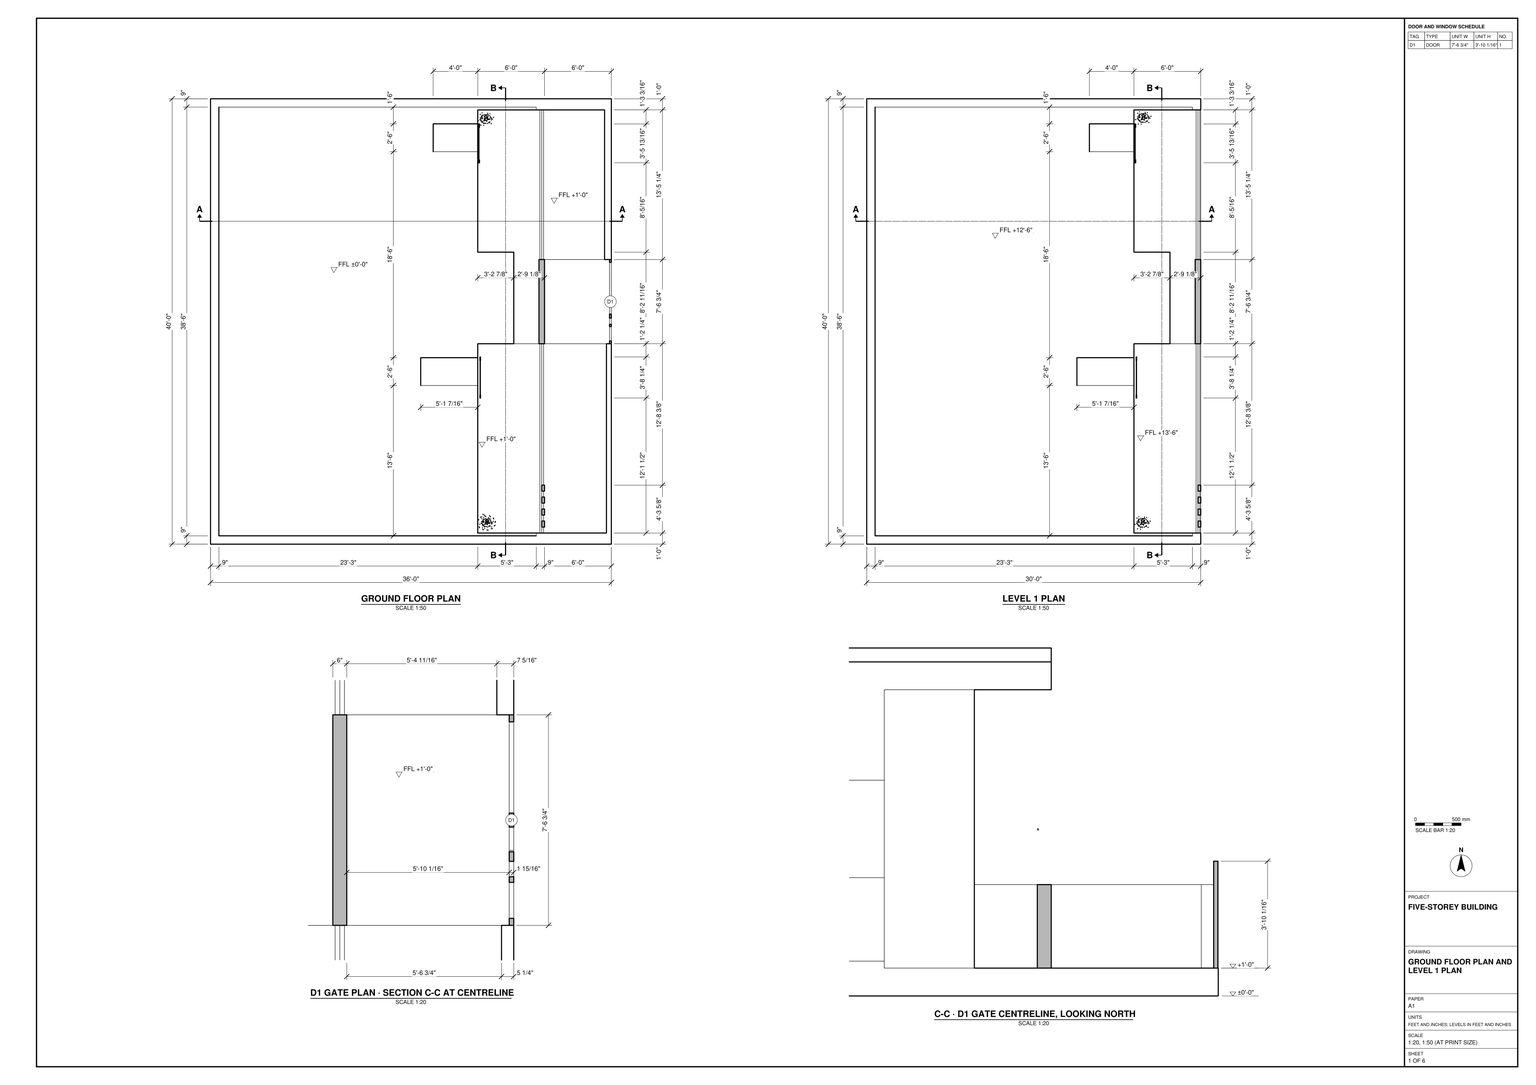
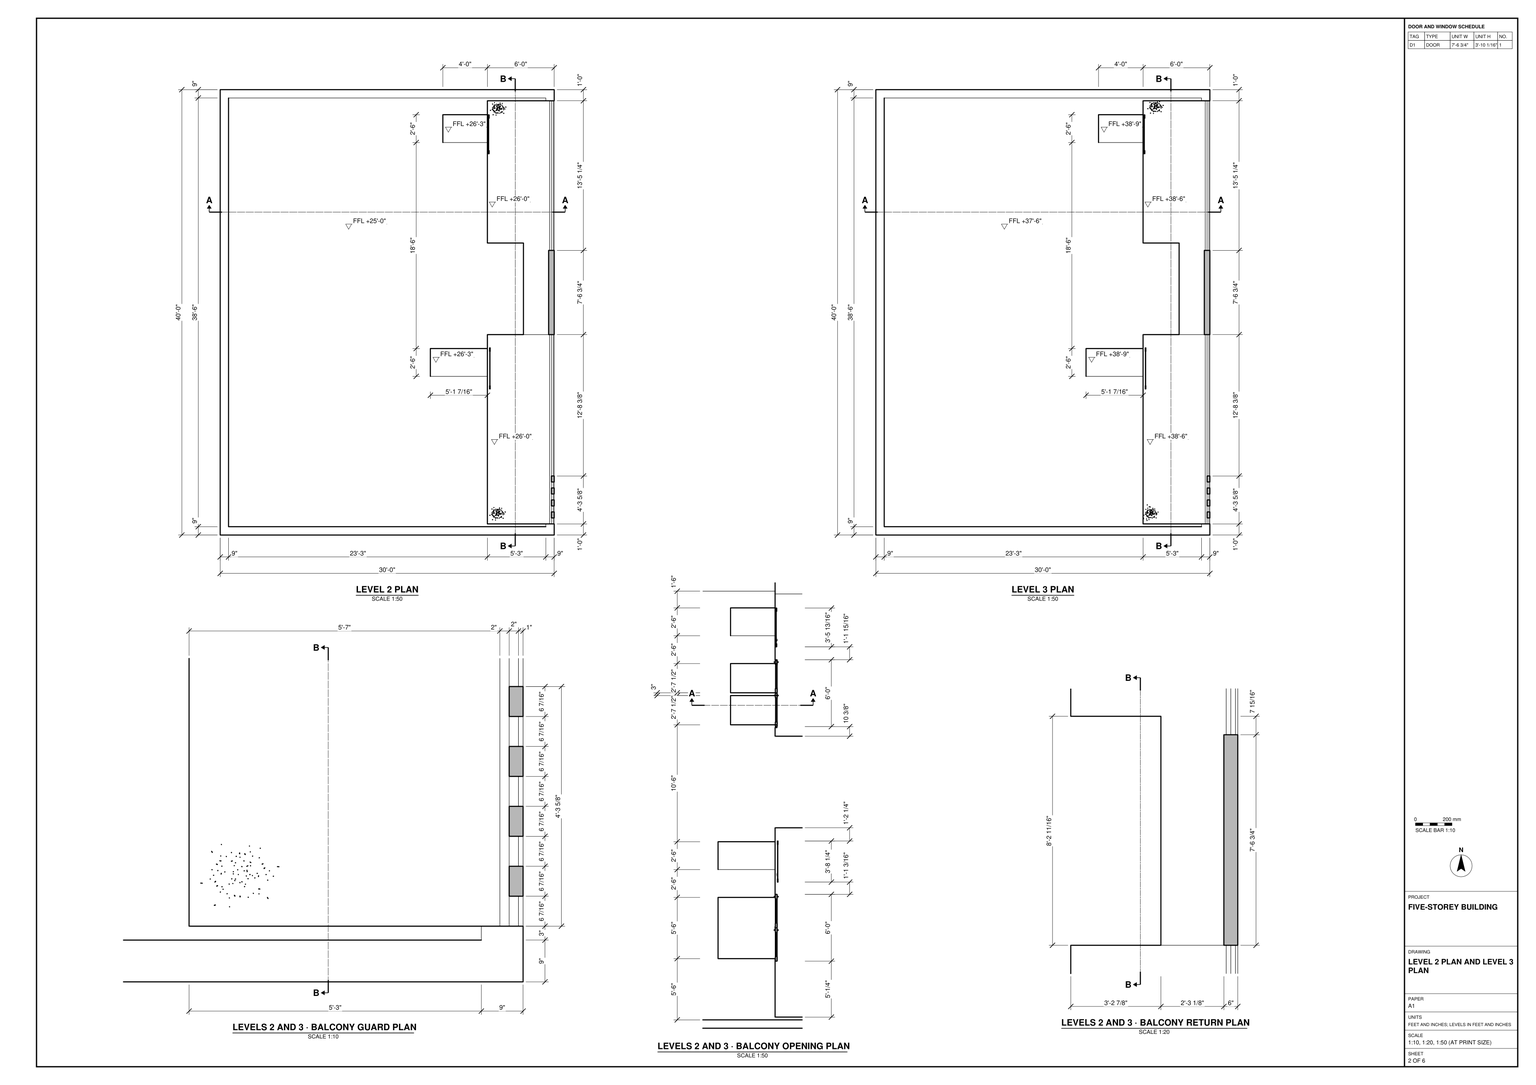
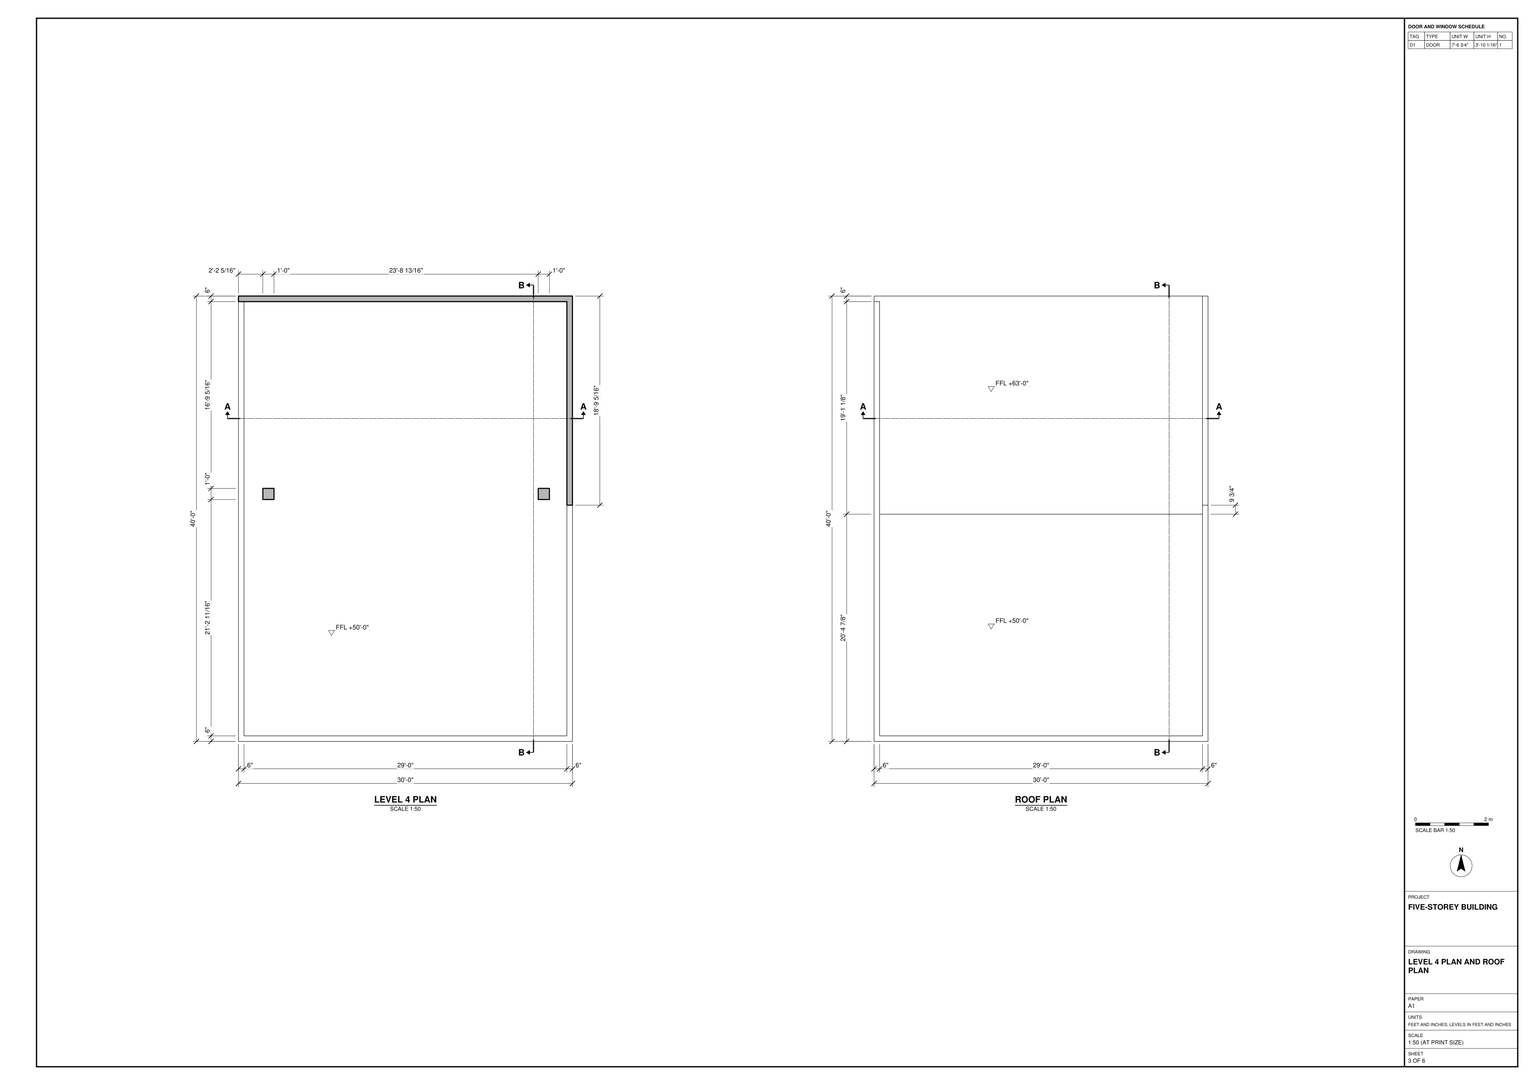
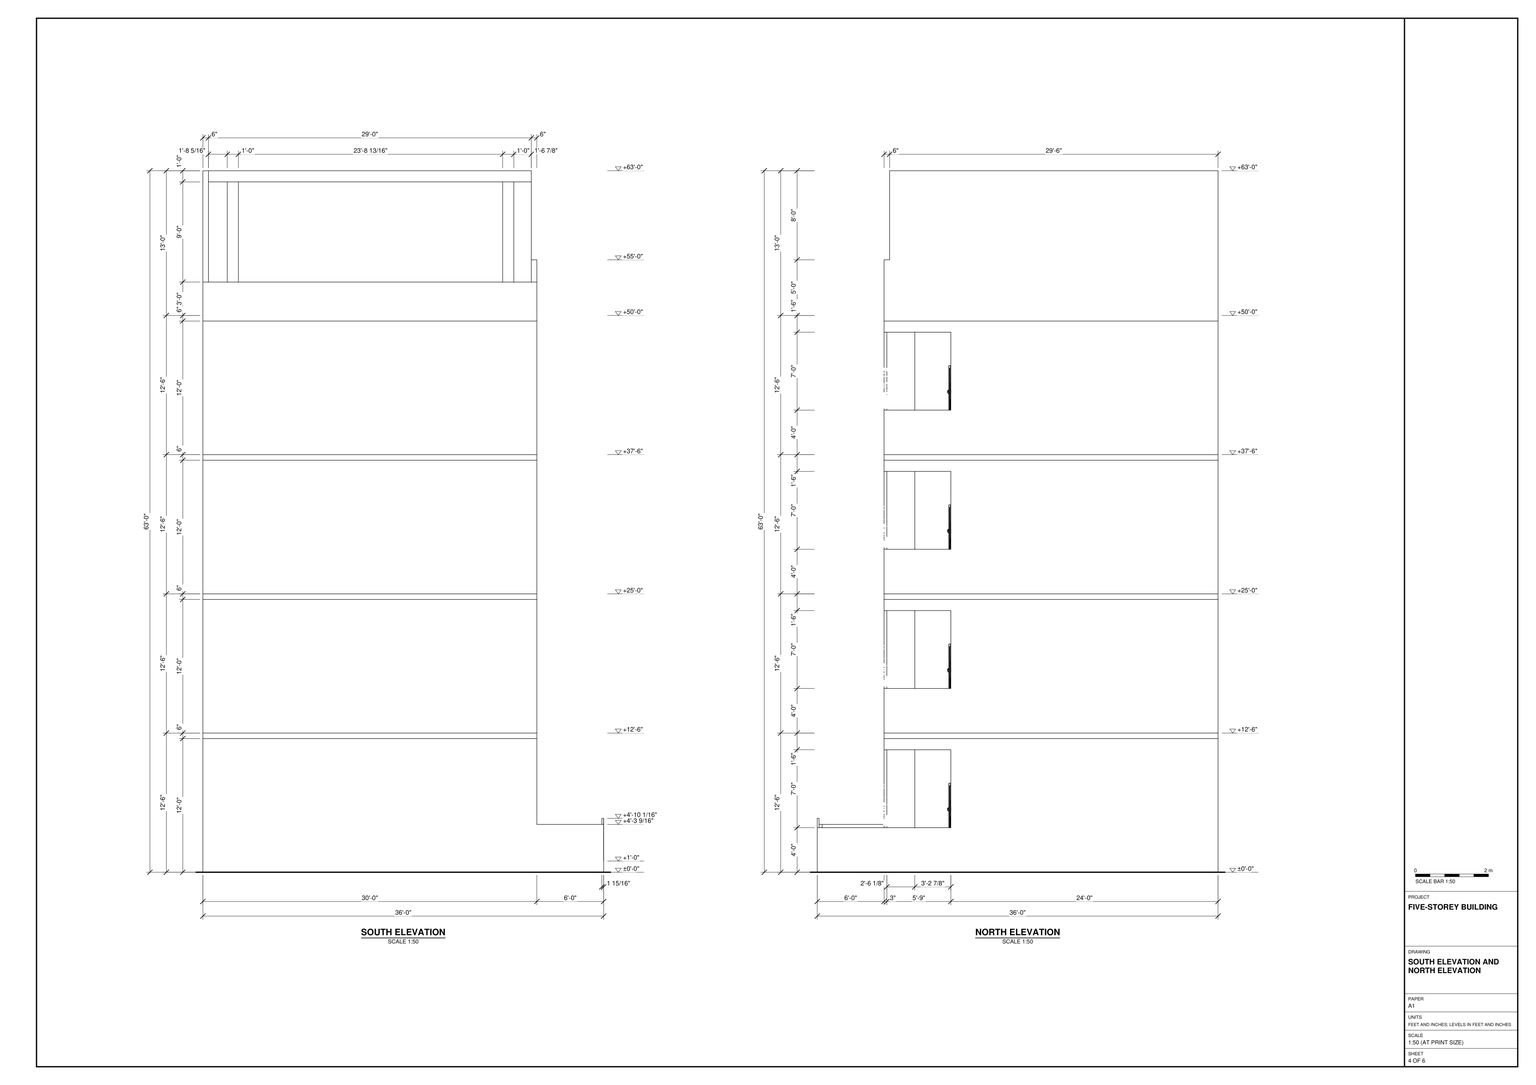
Build the five-storey building in SketchUp from task_files/diagram_01.pdf. Work in feet and inches. The model measures 36'-0" along X, 40'-0" along Y and 63'-0" in height. Set the storey levels to ±0'-0", +12'-6", +25'-0", +37'-6" and +50'-0".

Lay out the rectangular ground floor with the raised strip along its east edge. Fit the entrance gate in the break in the outer wall of this strip, using the gate plan and section for its size and position. Set the upper floors back from the gate side to give them a width of 30'-0" while retaining the full depth. Model the floor slabs, wall thicknesses and openings as drawn. Follow the balcony plans for the changes in floor height, the wider end portions and the narrow connecting portion. Include the guard members, returns and planting at the ends shown on the plans.

At +50'-0", distinguish the open terrace from the portion under the higher roof. Model the perimeter edges, walls and square supports in their drawn positions. Decor and loose items, including plants, may be any suitable library components.

Keep the walls, slabs and roof as separate groups or components, and group each furniture or joinery piece separately where shown. Use components for repeated parts. Save one SketchUp model as output_files/five_storey_building_stepped_balconies_and_roof_terrace.skp.

# SketchUp Ruby script. Lengths in inches.
U = 1.inch
M = Sketchup.active_model
def pt(a) = Geom::Point3d.new(a.map { |v| v * U })
def face(e, loops, mat)
  f = e.add_face(loops[0].map { |a| pt(a) })
  loops[1..].each { |l| e.add_face(l.map { |a| pt(a) }).erase! }
  f.material = f.back_material = mat if mat
  f
end
# faces: each face lists its corners as indices into pts; further lists are holes
def faces(e, pts, list, mat = nil) = list.each { |f| face(e, (f[0].is_a?(Array) ? f : [f]).map { |l| l.map { |i| pts[i] } }, mat) }
# xy, xz, yz: faces in a plane at the given z, y or x. An outline is a flat list of corners, or four numbers for a rectangle; further outlines are holes
def ring(l) = l.size == 4 ? [[l[0], l[1]], [l[2], l[1]], [l[2], l[3]], [l[0], l[3]]] : l.each_slice(2).to_a
def flat(e, list, mat, &to3) = list.each { |f| face(e, (f[0].is_a?(Array) ? f : [f]).map { |l| ring(l).map { |u, v| to3.(u, v) } }, mat) }
def xy(e, z, list, mat = nil) = flat(e, list, mat) { |x, y| [x, y, z] }
def xz(e, y, list, mat = nil) = flat(e, list, mat) { |x, z| [x, y, z] }
def yz(e, x, list, mat = nil) = flat(e, list, mat) { |y, z| [x, y, z] }
def lines(e, pts, list) = list.each { |a, b| e.add_line(pt(pts[a]), pt(pts[b])) }
# prism: a flat outline (further loops are holes) pulled along v
def prism(e, loops, v, mat = nil)
  f = face(e, loops, mat); d = Geom::Vector3d.new(v.map { |x| x * U })
  f.pushpull(f.normal.samedirection?(d) ? d.length : -d.length)
end
def box(e, o, s, mat = nil) = prism(e, [[o, [o[0] + s[0], o[1], o[2]], [o[0] + s[0], o[1] + s[1], o[2]], [o[0], o[1] + s[1], o[2]]]], [0, 0, s[2]], mat)
def at(x, y, z, deg = 0) = Geom::Transformation.translation(pt([x, y, z])) * Geom::Transformation.rotation(ORIGIN, Z_AXIS, deg.degrees)
def axes(o, x, y, z) = Geom::Transformation.new([*x, 0, *y, 0, *z, 0, *pt(o).to_a, 1])
def part(name) = M.definitions.add(name)
# library, detail: a bought-in or finely detailed component or shape, given as its bounding box
def library(name, o, s) = part(name).tap { |d| box(d.entities, o, s) }
def detail(e, o, s) = box(e.add_group.entities, o, s)
def put(e, d, t, mat = nil) = e.add_instance(d, t).tap { |i| i.material = mat if mat }
def group(e, t, mat = nil) = e.add_group.tap { |g| g.transformation = t; g.material = mat if mat }.entities
root = M.entities
M.materials.add("B01_Ivory_Dust").color = [255, 217, 206]
M.materials.add("C01_Vanilla_Cream").color = [244, 228, 212]
M.materials.add("LightPink_Translucent").color = [144, 107, 117]
c1 = library("Double casement window",[0,0,0],[5.02,56.42,60])
c2 = part("blade")
p = [[2.15,0.21,22],[0,0.17,0],[0.09,0.45,0],[2.18,0.31,22],[2.29,0.31,22],[0.38,0.45,0],
  [2.48,0.24,33],[2.49,0.24,33],[2.48,0.22,33]]
faces(c2.entities,p,[[0,1,2,3],[4,5,2,3],[6,3,4,7],[8,0,3,6]])
c3 = part("seeds")
p = [[0.3,-0.1,1.38],[-0.01,-0.03,1.59],[-0.01,-0.03,0.03],[0.14,-0.07,-0.07],[0.29,-0.03,3],[0.15,0.01,3.11]]
faces(c3.entities,p,[[0,1,2,3],[1,0,4,5]],"LightPink_Translucent")
c4 = part("blade with seeds")
put(c4.entities,c2,at(0,0,0))
put(c4.entities,c3,axes([2.4,0.25,30.99],[1.5799,-0.05474,1.17369],[-0.12525,1.92788,0.29478],[-0.07173,-0.02425,1.56792]))
c5 = part("Regal mist grass")
put(c5.entities,c4,axes([-3.26,-3.84,1.05],[0.05632,0.08194,0.78597],[-0.27153,0.73654,-0.07427],[-0.27499,0.00533,0.13909]))
put(c5.entities,c4,axes([-3.73,-1.59,0.19],[0.48504,-0.05875,0.50893],[-0.30767,0.51765,0.37393],[-0.23969,-0.07765,0.1121]))
put(c5.entities,c4,axes([-2.85,-2.28,0.11],[0.14833,0.22859,0.63362],[-0.3418,0.62134,-0.13627],[-0.35096,-0.14851,0.27091]))
put(c5.entities,c4,axes([3.2,1.81,0.97],[0.43228,0.51405,-0.15691],[-0.49359,0.48662,0.20258],[0.25079,0.07404,0.38762]))
put(c5.entities,c4,axes([2.7,2.1,0.19],[-0.42777,-0.23608,0.50893],[0.55235,-0.23987,0.37393],[0.14898,0.20319,0.1121]))
put(c5.entities,c4,axes([2.71,1.87,1.19],[0.04068,-0.83498,-0.05388],[0.77022,0.02282,-0.29906],[0.29664,0.058,0.45442]))
put(c5.entities,c4,axes([-3.45,-1.04,0.97],[-0.63139,-0.22904,-0.15691],[0.18416,-0.66822,0.20258],[-0.25421,0.06127,0.38762]))
put(c5.entities,c4,axes([-0.36,0.56,0.04],[0.20136,-0.97289,-0.10381],[0.95476,0.16959,0.22717],[-0.16683,-0.13435,0.69317]))
put(c5.entities,c4,axes([-2.43,-0.5,0.06],[0,0.82104,0.22],[-0.85,0,0],[0,-0.187,0.69788]))
put(c5.entities,c4,axes([1.82,-1.29,-0.13],[0.7903,0.13461,-0.27628],[-0.16677,0.83032,-0.07251],[0.23585,0.10061,0.60984]))
put(c5.entities,c4,axes([2.42,-3.36,0.01],[0.475,-0.82272,0],[0.79469,0.45881,-0.22867],[0.181,0.1045,0.72539]))
put(c5.entities,c4,axes([-2,3.05,0.45],[0.01669,-0.42385,0.68389],[0.75077,0.22388,0.09451],[-0.06505,0.45172,0.32293]))
put(c5.entities,c4,axes([-0.36,3.06,1.2],[-0.74862,-0.21464,0.23609],[0.25599,-0.70567,0.19467],[0.04499,0.27751,0.48853]))
put(c5.entities,c4,axes([-0.35,2.54,1.2],[0.22904,-0.63139,0.15691],[0.66822,0.18416,-0.20258],[0.06127,0.25421,0.38762]))
put(c5.entities,c4,axes([0.87,-4.07,1.06],[0.74862,0.21464,0.21269],[-0.25599,0.70567,0.17538],[-0.04499,-0.27751,0.44012]))
put(c5.entities,c4,axes([0.86,-3.55,1.2],[-0.22904,0.63139,0.15691],[-0.66822,-0.18416,-0.20258],[-0.06127,-0.25421,0.38762]))
put(c5.entities,c4,axes([-2.31,3.6875,0.11],[0.23975,-0.12952,0.63362],[0.59193,0.39053,-0.13627],[-0.17618,0.33792,0.27091]))
put(c5.entities,c4,axes([-0.89,-5.97,1.05],[-0.01417,0.09841,0.78597],[-0.69904,0.35716,-0.07427],[-0.20571,-0.18257,0.13909]))
put(c5.entities,c4,axes([2.82,2.98,-0.38],[0.05535,-0.11853,0.78135],[0.69686,-0.3491,-0.11937],[0.21127,0.18068,0.13309]))
put(c5.entities,c4,axes([0.6,3.36,1.05],[0.00225,-0.0994,0.78597],[0.65107,-0.43855,-0.07427],[0.22615,0.15653,0.13909]))
put(c5.entities,c4,axes([3.04,1.81,1.06],[-0.56019,0.541,0.21269],[-0.48313,-0.57453,0.17538],[0.26282,0.09979,0.44012]))
put(c5.entities,c4,axes([2.59,1.54,1.2],[-0.43228,-0.51405,0.15691],[0.49359,-0.48662,-0.20258],[0.25079,0.07404,0.38762]))
put(c5.entities,c4,axes([2.85,-2.86,-0.15],[0.71104,0.41052,-0.22],[-0.425,0.73612,0],[0.16194,0.0935,0.69788]))
put(c5.entities,c4,axes([-3.85,-0.6,1.05],[-0.12406,0.1066,0.77516],[0.01055,0.77884,-0.12259],[-0.28438,0.10128,0.06217]))
put(c5.entities,c4,axes([1.3,0.61,0.12],[0.56129,0.4933,0.06416],[-0.46819,0.55654,-0.18321],[-0.13032,0.07524,0.56159]))
put(c5.entities,c4,axes([1.125,0.43,0.14],[0.08853,0.93685,-0.12892],[-0.92207,0.05665,-0.22156],[-0.16237,0.12479,0.70765]))
put(c5.entities,c4,axes([-0.48,-0.93,-0.06],[0.36861,-0.73982,-0.19823],[0.76592,0.35605,0.0954],[0,-0.17054,0.63647]))
put(c5.entities,c4,axes([-3.05,-1.34,1.19],[0.38226,0.74345,-0.05388],[-0.67844,0.36535,-0.29906],[-0.2859,0.09809,0.45442]))
put(c5.entities,c4,axes([-0.85,-4.05,1.06],[0.3453,-0.52156,0.02849],[0.49172,0.30366,0.2243],[-0.15897,-0.16722,0.34202]))
put(c5.entities,c4,axes([-0.91,-3.46,1.17],[-0.64782,-0.39685,-0.31479],[0.4604,-0.69542,0.03799],[-0.23471,-0.23695,0.44531]))
put(c5.entities,c4,axes([5.64,-0.84,1.05],[0.10543,-0.12506,0.77516],[-0.13494,-0.76713,-0.12259],[0.26452,-0.14545,0.06217]))
put(c5.entities,c4,axes([0.86,-0.73,-0.0625],[0,-0.95,0],[0.95,0,0],[0,0,0.79515]))
put(c5.entities,c4,axes([1.65,0.49,0.68],[-0.2822,-0.14146,0.75935],[0.58401,-0.59344,0.0614],[0.36399,0.26771,0.32462]))
put(c5.entities,c4,axes([3.38,1.37,1.05],[0.16298,-0.01389,0.77516],[0.44703,-0.63786,-0.12259],[0.28989,0.0842,0.06217]))
put(c5.entities,c4,axes([3.82,0.11,1.06],[-0.21464,0.74862,0.21269],[-0.70567,-0.25599,0.17538],[0.27751,-0.04499,0.44012]))
put(c5.entities,c4,axes([3.3,0.1,1.2],[-0.63139,-0.22904,0.15691],[0.18416,-0.66822,-0.20258],[0.25421,-0.06127,0.38762]))
put(c5.entities,c4,axes([0.07,2.77,1.03],[0.74683,0.20582,-0.22641],[-0.25599,0.70567,-0.17538],[0.06848,0.28411,0.43322]))
put(c5.entities,c4,axes([-0.56,3.11,1.06],[-0.55982,0.27904,0.02849],[-0.27401,-0.50883,0.2243],[0.05406,0.2243,0.34202]))
put(c5.entities,c4,axes([-0.21,2.64,1.17],[0.36261,0.66759,-0.31479],[-0.74642,0.37205,0.03799],[0.08479,0.32256,0.44531]))
put(c5.entities,c4,axes([0.99,-1.65,0.12],[0.14656,-0.73274,0.06416],[0.71607,0.12719,-0.18321],[0.13032,0.07524,0.56159]))
put(c5.entities,c4,axes([1.74,-2.51,0.06],[-0.81639,0.21792,0.07817],[-0.20159,-0.81098,0.15546],[0.07281,0.11816,0.71074]))
put(c5.entities,c4,axes([1.48,-0.78,0.16],[0.36861,-0.73982,0.19823],[0.76592,0.35605,-0.0954],[0,0.17054,0.63647]))
put(c5.entities,c4,axes([0.64,1.03,0.43],[0.65653,0.33108,0.67022],[-0.64318,0.71325,0.26504],[-0.28809,-0.42273,0.56186]))
put(c5.entities,c4,axes([-3.14,0.74,1.06],[-0.18842,-0.75564,0.21269],[0.73912,-0.13114,0.17538],[-0.21784,0.17772,0.44012]))
put(c5.entities,c4,axes([-3.22,0.89,0.97],[-0.66132,0.11734,-0.15691],[-0.17463,-0.67077,0.20258],[-0.18951,0.18017,0.38762]))
put(c5.entities,c4,axes([-2.23,-2.48,1.17],[-0.75946,-0.01977,-0.31479],[0.05101,-0.83245,0.03799],[-0.32174,-0.08785,0.44531]))
put(c5.entities,c4,axes([-2.76,-3.02,1.22],[0.62742,-0.60592,0.23822],[0.54111,0.64347,0.19642],[-0.29436,-0.11177,0.49293]))
put(c5.entities,c4,axes([-2.08,-2.56,1.2],[0.43228,0.51405,0.15691],[-0.49359,0.48662,-0.20258],[-0.25079,-0.07404,0.38762]))
put(c5.entities,c4,axes([1.55,-0.55,0.14],[0.8556,0.39175,-0.12892],[-0.41198,0.82685,-0.22156],[0.02689,0.20301,0.70765]))
put(c5.entities,c4,axes([1.48,-0.16,-0.06],[0.53033,0.53033,0],[-0.53033,0.53033,0],[0,0,0.75]))
put(c5.entities,c4,axes([2.63,-2.96,1.19],[-0.83498,-0.04068,-0.05388],[0.02282,-0.77022,-0.29906],[0.058,-0.29664,0.45442]))
put(c5.entities,c4,axes([2.0625,-3.25,1.03],[-0.54387,-0.55166,-0.22641],[0.57453,-0.48313,-0.17538],[0.08275,-0.28029,0.43322]))
put(c5.entities,c4,axes([3.97,0.02,0.97],[0.63139,0.22904,-0.15691],[-0.18416,0.66822,0.20258],[0.25421,-0.06127,0.38762]))
put(c5.entities,c4,axes([4.49,1.89,0.7],[-0.14541,-0.69018,-0.01547],[0.68728,-0.15867,-0.07015],[0.14352,0.04375,0.23137]))
put(c5.entities,c4,axes([3.57,0.32,1.19],[-0.38226,-0.74345,-0.05388],[0.67844,-0.36535,-0.29906],[0.2859,-0.09809,0.45442]))
put(c5.entities,c4,axes([-1.14,-3.99,0.97],[-0.11734,-0.66132,-0.15691],[0.67077,-0.17463,0.20258],[-0.18017,-0.18951,0.38762]))
put(c5.entities,c4,axes([-0.04,-4.56,-0.1],[-0.52501,0.47102,-0.01725],[-0.48105,-0.51587,-0.0782],[-0.03387,-0.14617,0.25794]))
put(c5.entities,c4,axes([-0.69,-4.1,1.37],[-0.50704,0.78711,-0.06035],[-0.7343,-0.45346,-0.33495],[-0.25525,-0.22238,0.50895]))
put(c5.entities,c4,axes([-1.22,-3.44,1.03],[-0.74969,0.19517,-0.22641],[-0.13114,-0.73912,-0.17538],[-0.20136,-0.21181,0.43322]))
put(c5.entities,c4,axes([3.39,-4.18,1.05],[-0.00733,-0.1634,0.77516],[-0.61941,-0.47227,-0.12259],[0.09577,-0.28628,0.06217]))
put(c5.entities,c4,axes([-2.27,-0.88,-0.01],[-0.70668,0.69027,0.13628],[-0.70711,-0.68301,-0.16169],[-0.02468,-0.19603,0.73059]))
put(c5.entities,c4,axes([-0.42,0.16,-0.06],[-0.4564,-0.68913,-0.19823],[0.69131,-0.48528,0.0954],[-0.14769,-0.08527,0.63647]))
put(c5.entities,c4,axes([-1.79,1.83,1.2],[0.51405,-0.43228,0.15691],[0.48662,0.49359,-0.20258],[-0.07404,0.25079,0.38762]))
put(c5.entities,c4,axes([-2.14,3.0625,0.21],[0.69018,-0.14539,0.02883],[0.15867,0.58575,-0.38241],[-0.04375,0.29652,0.34277]))
put(c5.entities,c4,axes([-0.57,2.8,1.19],[0.74345,-0.38226,-0.05388],[0.36535,0.67844,-0.29906],[0.09809,0.2859,0.45442]))
put(c5.entities,c4,axes([-2.68,0.49,1.2],[0.66132,-0.11734,0.15691],[0.17463,0.67077,-0.20258],[-0.18951,0.18017,0.38762]))
put(c5.entities,c4,axes([-2.06,2.27,1.06],[-0.541,-0.56019,0.21269],[0.57453,-0.48313,0.17538],[-0.09979,0.26282,0.44012]))
put(c5.entities,c4,axes([1.29,-3.38,0.68],[-0.14146,0.2822,0.75935],[-0.59344,-0.58401,0.0614],[0.26771,-0.36399,0.32462]))
put(c5.entities,c4,axes([3.8,-1.61,1.06],[0.52156,0.3453,0.02849],[-0.30366,0.49172,0.2243],[0.16722,-0.15897,0.34202]))
put(c5.entities,c4,axes([3.21,-1.68,1.17],[0.39685,-0.64782,-0.31479],[0.69542,0.4604,0.03799],[0.23695,-0.23471,0.44531]))
put(c5.entities,c4,axes([4.29,-0.11,-0.16],[-0.48932,0.09853,0.62734],[-0.07789,-0.78429,0.03591],[0.34272,-0.11871,0.35698]))
put(c5.entities,c4,axes([-0.57,-0.3125,0.14],[-0.8556,-0.39175,-0.12892],[0.41198,-0.82685,-0.22156],[-0.02689,-0.20301,0.70765]))
put(c5.entities,c4,axes([-3.375,-0.75,-0.38],[0.01927,0.12939,0.78135],[-0.38842,0.67573,-0.11937],[-0.2759,-0.03406,0.13309]))
put(c5.entities,c4,axes([-3.83,2.3125,1.05],[-0.01889,0.16248,0.77516],[0.53593,0.56522,-0.12259],[-0.1403,0.26729,0.06217]))
put(c5.entities,c4,axes([-5.23,0.19,1.05],[0.09696,0.02202,0.78597],[0.29994,0.72543,-0.07427],[-0.19848,0.1904,0.13909]))
put(c5.entities,c4,axes([-1.08,-3.5625,0.01],[-0.475,-0.82272,0],[0.79469,-0.45881,-0.22867],[0.181,-0.1045,0.72539]))
put(c5.entities,c4,axes([-0.27,-3.37,-0.14],[0.70879,0.20315,-0.13726],[-0.17846,0.71541,0.13726],[0.14289,-0.0825,0.61578]))
put(c5.entities,c4,axes([3.53,-0.32,1.03],[0.20582,-0.74683,-0.22641],[0.70567,0.25599,-0.17538],[0.28411,-0.06848,0.43322]))
put(c5.entities,c4,axes([2.25,-0.8,0.68],[-0.31513,0.0186,0.75935],[0.20905,-0.80594,0.0614],[0.44908,0.04985,0.32462]))
put(c5.entities,c4,axes([3.875,0.31,1.06],[0.27904,0.55982,0.02849],[-0.50883,0.27401,0.2243],[0.2243,-0.05406,0.34202]))
put(c5.entities,c4,axes([3.4,-0.04,1.17],[0.66759,-0.36261,-0.31479],[0.37205,0.74642,0.03799],[0.32256,-0.08479,0.44531]))
put(c5.entities,c4,axes([-2.2,-2.88,1.19],[-0.04068,0.83498,-0.05388],[-0.77022,-0.02282,-0.29906],[-0.29664,-0.058,0.45442]))
put(c5.entities,c4,axes([-2.49,-2.3125,1.03],[-0.55166,0.54387,-0.22641],[-0.48313,-0.57453,-0.17538],[-0.28029,-0.08275,0.43322]))
put(c5.entities,c4,axes([0.49,1.3125,0.68],[-0.17367,-0.26361,0.75935],[0.80249,-0.22193,0.0614],[0.18137,0.41384,0.32462]))
put(c5.entities,c4,axes([-2.47,-3.02,1.06],[0.03826,-0.62433,0.02849],[0.57767,0.01712,0.2243],[-0.22128,-0.06533,0.34202]))
put(c5.entities,c4,axes([0.09,-5.13,-0.38],[-0.12743,0.02958,0.78135],[-0.70471,-0.33298,-0.11937],[0.01182,-0.27774,0.13309]))
put(c5.entities,c4,axes([1.8,-0.61,0.12],[0.70785,-0.23944,0.06416],[0.24789,0.68373,-0.18321],[0,0.15048,0.56159]))
put(c5.entities,c4,axes([2.92,-0.39,0.06],[-0.59691,-0.59805,0.07817],[0.60154,-0.58007,0.15546],[-0.06593,0.12214,0.71074]))
put(c5.entities,c4,axes([2.77,-3.23,1.06],[0.62433,0.03826,0.02849],[-0.01712,0.57767,0.2243],[0.06533,-0.22128,0.34202]))
put(c5.entities,c4,axes([-0.93,1.44,0.68],[-0.0186,-0.31513,0.75935],[0.80594,0.20905,0.0614],[-0.04985,0.44908,0.32462]))
put(c5.entities,c4,axes([2.23,-3,1.17],[0.01977,-0.75946,-0.31479],[0.83245,0.05101,0.03799],[0.08785,-0.32174,0.44531]))
put(c5.entities,c4,axes([-2.22,0.85,0.68],[0.14146,-0.2822,0.75935],[0.59344,0.58401,0.0614],[-0.26771,0.36399,0.32462]))
put(c5.entities,c4,axes([2.57,-3.29,1.06],[0.541,0.56019,0.21269],[-0.57453,0.48313,0.17538],[0.09979,-0.26282,0.44012]))
put(c5.entities,c4,axes([-0.83,0.43,-0.13],[-0.7903,-0.13461,-0.27628],[0.16677,-0.83032,-0.07251],[-0.23585,-0.10061,0.60984]))
put(c5.entities,c4,axes([1.17,1.85,0.11],[0.01341,-0.27217,0.63362],[0.64069,-0.30401,-0.13627],[0.19778,0.32575,0.27091]))
put(c5.entities,c4,axes([-3.05,-0.3125,0.68],[0.26361,-0.17367,0.75935],[0.22193,0.80249,0.0614],[-0.41384,0.18137,0.32462]))
put(c5.entities,c4,axes([0.55,4.79,1.46],[0.52501,-0.47102,-0.02875],[0.48105,0.51587,-0.13034],[0.03387,0.14617,0.4299]))
put(c5.entities,c4,axes([1.19,2.78,1.19],[0.45272,-0.70277,-0.05388],[0.65562,0.40488,-0.29906],[0.2279,0.19855,0.45442]))
put(c5.entities,c4,axes([3.41,0.38,-0.14],[-0.53033,0.51226,-0.13726],[-0.53033,-0.51226,0.13726],[0,0.165,0.61578]))
put(c5.entities,c4,axes([1.4,-1.03,-0.06],[0.4564,0.68913,-0.19823],[-0.69131,0.48528,0.0954],[0.14769,0.08527,0.63647]))
put(c5.entities,c4,axes([-4.42,2.5,0.19],[0.31662,-0.37211,0.50893],[0.12494,0.58908,0.37393],[-0.22881,0.10548,0.1121]))
put(c5.entities,c4,axes([2.01,-2.93,0.06],[-0.71104,-0.41052,0.22],[0.425,-0.73612,0],[0.16194,0.0935,0.69788]))
put(c5.entities,c4,axes([-2.08,0.23,0.68],[0.18976,-0.25227,0.75935],[0.47913,0.68094,0.0614],[-0.32863,0.3101,0.32462]))
put(c5.entities,c4,axes([-3.03,0.43,1.19],[0.70277,0.45272,-0.05388],[-0.40488,0.65562,-0.29906],[-0.19855,0.2279,0.45442]))
put(c5.entities,c4,axes([1.41,2.83,-0.15],[-0.71104,0.41052,-0.22],[-0.425,-0.73612,0],[-0.16194,0.0935,0.69788]))
put(c5.entities,c4,axes([0.92,0.8,0.05],[-0.74186,-0.66083,-0.11162],[0.62425,-0.74205,0.24427],[-0.19977,0.0773,0.74534]))
put(c5.entities,c4,axes([1.1,0,-0.02],[-0.70668,-0.70668,-0.02717],[0.70711,-0.70711,0],[-0.02468,-0.02468,0.77794]))
put(c5.entities,c4,axes([-2.8,-1.26,-0.15],[0,-0.82104,-0.22],[0.85,0,0],[0,-0.187,0.69788]))
put(c5.entities,c4,axes([1.34,-0.35,-0.02],[0,0.94953,-0.02498],[-0.95,0,0],[0,0.02984,0.79476]))
put(c5.entities,c4,axes([2.98,2.01,1.06],[-0.03826,0.62433,0.02849],[-0.57767,-0.01712,0.2243],[0.22128,0.06533,0.34202]))
put(c5.entities,c4,axes([-1.42,-3.85,0.68],[0.17367,0.26361,0.75935],[-0.80249,0.22193,0.0614],[-0.18137,-0.41384,0.32462]))
put(c5.entities,c4,axes([2.75,1.47,1.17],[0.75946,0.01977,-0.31479],[-0.05101,0.83245,0.03799],[0.32174,0.08785,0.44531]))
put(c5.entities,c4,axes([-0.4375,2.95,-0.38],[0.12296,-0.04468,0.78135],[0.7396,0.2459,-0.11937],[0.02163,0.27715,0.13309]))
put(c5.entities,c4,axes([1.25,2.43,1.2],[-0.11734,-0.66132,0.15691],[0.67077,-0.17463,-0.20258],[0.18017,0.18951,0.38762]))
put(c5.entities,c4,axes([1.46,2.61,-0.07],[-0.46908,-0.8256,-0.02278],[0.79469,-0.45881,0.22867],[-0.19583,0.0786,0.72503]))
put(c5.entities,c4,axes([1.48,2.1875,-0.01],[0.95113,0.26686,0.13628],[-0.23795,0.95388,-0.16169],[-0.15742,0.11938,0.73059]))
put(c5.entities,c4,axes([1.71,-1.37,0.94],[-0.65649,-0.4266,0.61271],[0.6932,-0.66419,0.26437],[0.21181,0.40027,0.59225]))
put(c5.entities,c4,axes([3.61,0.25,-0.07],[-0.94953,-0.00656,-0.02205],[0,-0.91763,0.22129],[-0.02984,0.20889,0.70164]))
put(c5.entities,c4,axes([-1.67,1.69,-0.14],[-0.17846,-0.71541,-0.13726],[0.70879,-0.20315,0.13726],[-0.14289,-0.0825,0.61578]))
put(c5.entities,c4,axes([-2.12,1.95,1.35],[0.83498,0.04068,-0.05981],[-0.02282,0.77022,-0.33196],[-0.058,0.29664,0.5044]))
put(c5.entities,c4,axes([-3.28,0.6,1.06],[-0.52156,-0.3453,0.02849],[0.30366,-0.49172,0.2243],[-0.16722,0.15897,0.34202]))
put(c5.entities,c4,axes([-2.68,0.97,1.03],[0.19517,0.74969,-0.22641],[-0.73912,0.13114,-0.17538],[-0.21181,0.20136,0.43322]))
put(c5.entities,c4,axes([-3.02,-0.7,1.03],[-0.20582,0.74683,-0.22641],[-0.70567,-0.25599,-0.17538],[-0.28411,0.06848,0.43322]))
put(c5.entities,c4,axes([-0.75,4.32,1.05],[0.0963,0.13221,0.77516],[0.77718,0.05194,-0.12259],[0.07815,0.29158,0.06217]))
put(c5.entities,c4,axes([-0.25,0.09,0.01],[0.96024,0.17298,0.20273],[-0.19542,0.97698,0.07956],[-0.14033,-0.09434,0.70387]))
put(c5.entities,c4,axes([3.41,-0.36,0.06],[0,-0.82104,0.22],[0.85,0,0],[0,0.187,0.69788]))
put(c5.entities,c4,axes([1.46,0.0625,-0.06],[-0.36861,0.73982,-0.19823],[-0.76592,-0.35605,0.0954],[0,0.17054,0.63647]))
put(c5.entities,c4,axes([-2.58,-3.03,0.68],[0.2822,0.14146,0.75935],[-0.58401,0.59344,0.0614],[-0.36399,-0.26771,0.32462]))
put(c5.entities,c4,axes([5.27,-1.64,1.05],[-0.09923,-0.00624,0.78597],[-0.41207,-0.66814,-0.07427],[0.16548,-0.21969,0.13909]))
put(c5.entities,c4,axes([-1.55,2.24,1.18],[0.54387,0.55166,-0.25132],[-0.57453,0.48313,-0.19467],[-0.08275,0.28029,0.48087]))
put(c5.entities,c4,axes([-2.06,2.44,0.97],[-0.51405,0.43228,-0.15691],[-0.48662,-0.49359,0.20258],[-0.07404,0.25079,0.38762]))
put(c5.entities,c4,axes([-1.87,2,-0.15],[-0.71104,-0.41052,-0.22],[0.425,-0.73612,0],[-0.16194,-0.0935,0.69788]))
put(c5.entities,c4,axes([5.09,2.53,1.05],[-0.0687,-0.07188,0.78597],[0.15027,-0.77048,-0.07427],[0.2706,-0.04923,0.13909]))
put(c5.entities,c4,axes([0.88,1.48,-0.02],[0.33031,0.94323,-0.02664],[-0.9438,0.33051,0],[0.01153,0.03294,0.76288]))
put(c5.entities,c4,axes([1.39,1.36,-0.07],[0.79762,-0.27858,-0.08506],[0.28027,0.80246,0.00004],[0.08804,-0.03079,0.77052]))
put(c5.entities,c4,axes([5.31,0.16,0.19],[-0.46941,0.13554,0.50893],[0.22095,-0.56018,0.37393],[0.24902,0.03833,0.1121]))
put(c5.entities,c4,axes([0.46,1.46,-0.0625],[-0.24789,-0.70785,0],[0.70785,-0.24789,0],[0,0,0.684]))
put(c5.entities,c4,axes([1.71,-4.23,0.11],[-0.21596,0.16619,0.63362],[-0.64676,-0.29087,-0.13627],[0.11989,-0.36174,0.27091]))
put(c5.entities,c4,axes([1.16,1.79,-0.0625],[0.76592,0.36861,0],[-0.36861,0.76592,0],[0,0,0.7752]))
put(c5.entities,c4,axes([3.79,-2.27,0.11],[-0.27141,-0.02432,0.63362],[-0.27805,-0.65237,-0.13627],[0.33343,-0.18455,0.27091]))
put(c5.entities,c4,axes([4.82,-0.62,-0.38],[-0.03971,-0.12465,0.78135],[0.27539,-0.72914,-0.11937],[0.27779,-0.01049,0.13309]))
put(c5.entities,c4,axes([1.09,-3.82,1.19],[-0.74345,0.38226,-0.05388],[-0.36535,-0.67844,-0.29906],[-0.09809,-0.2859,0.45442]))
put(c5.entities,c4,axes([0.45,-3.79,1.03],[-0.74683,-0.20582,-0.22641],[0.25599,-0.70567,-0.17538],[-0.06848,-0.28411,0.43322]))
put(c5.entities,c4,axes([1.07,-4.125,1.06],[0.55982,-0.27904,0.02849],[0.27401,0.50883,0.2243],[-0.05406,-0.2243,0.34202]))
put(c5.entities,c4,axes([0.72,-3.65,1.17],[-0.36261,-0.66759,-0.31479],[0.74642,-0.37205,0.03799],[-0.08479,-0.32256,0.44531]))
put(c5.entities,c4,axes([0.55,0.66,-0.06],[-0.82501,0.05068,-0.19823],[-0.07461,-0.84133,0.0954],[-0.14769,0.08527,0.63647]))
put(c5.entities,c4,axes([-1.4375,2.49,0.01],[-0.475,0.82272,0],[-0.79469,-0.45881,-0.22867],[-0.181,-0.1045,0.72539]))
put(c5.entities,c4,axes([2.06,2.7,0.01],[0.475,0.82272,0],[-0.79469,0.45881,-0.22867],[-0.181,0.1045,0.72539]))
put(c5.entities,c4,axes([1.25,2.5,-0.14],[-0.70879,-0.20315,-0.13726],[0.17846,-0.71541,0.13726],[-0.14289,0.0825,0.61578]))
put(c5.entities,c4,axes([-4.18,2.4,1.46],[0.67042,0.21916,-0.02875],[-0.20623,0.67454,-0.13034],[-0.10965,0.10242,0.4299]))
put(c5.entities,c4,axes([-1.87,-4.98,0.19],[0.39631,0.28576,0.50893],[-0.57716,0.17178,0.37393],[-0.12349,-0.21962,0.1121]))
put(c5.entities,c4,axes([-1.64,-4.54,0.11],[-0.04601,0.26859,0.63362],[-0.67257,0.22484,-0.13627],[-0.15721,-0.34715,0.27091]))
put(c5.entities,c4,axes([-3.36,-1.32,1.06],[-0.27904,-0.55982,0.02849],[0.50883,-0.27401,0.2243],[-0.2243,0.05406,0.34202]))
put(c5.entities,c4,axes([-0.3,-1.11,0.16],[-0.82501,0.05068,0.19823],[-0.07461,-0.84133,-0.0954],[0.14769,-0.08527,0.63647]))
put(c5.entities,c4,axes([0.41,-1.33,0.01],[-0.62993,0.7451,0.20273],[-0.74838,-0.65773,0.07956],[0.15186,-0.07436,0.70387]))
put(c5.entities,c4,axes([0.41,-2.01,-0.13],[0.51173,-0.61712,-0.27628],[0.63569,0.55959,-0.07251],[0.20505,-0.15394,0.60984]))
put(c5.entities,c4,axes([-1.53,-1.15,0.44],[0.21595,-0.11877,0.78455],[0.07447,0.82927,0.0614],[-0.46776,0.11004,0.2804]))
put(c5.entities,c4,axes([1.65,-0.55,0.22],[-0.02075,-0.77304,0.62596],[0.93928,0.20038,0.26504],[-0.22215,0.423,0.59086]))
put(c5.entities,c4,axes([-0.15,-1.29,0.14],[-0.08853,-0.93685,-0.12892],[0.92207,-0.05665,-0.22156],[0.16237,-0.12479,0.70765]))
put(c5.entities,c4,axes([-0.43,-3.69,-0.15],[0.71104,-0.41052,-0.22],[0.425,0.73612,0],[0.16194,-0.0935,0.69788]))
put(c5.entities,c4,axes([5.18,-0.8,-0.04],[-0.47102,-0.52501,-0.02875],[0.51587,-0.48105,-0.13034],[0.14617,-0.03387,0.4299]))
put(c5.entities,c4,axes([3.54,-1.44,1.19],[-0.70277,-0.45272,-0.05388],[0.40488,-0.65562,-0.29906],[0.19855,-0.2279,0.45442]))
put(c5.entities,c4,axes([3.19,-1.98,1.03],[-0.19517,-0.74969,-0.22641],[0.73912,-0.13114,-0.17538],[0.21181,-0.20136,0.43322]))
put(c5.entities,c4,axes([4.43,1.06,0.11],[-0.18297,-0.20193,0.63362],[0.23807,-0.668,-0.13627],[0.37019,0.09049,0.27091]))
put(c5.entities,c4,axes([3.74,-1.9,0.97],[0.66132,-0.11734,-0.15691],[0.17463,0.67077,0.20258],[0.18951,-0.18017,0.38762]))
put(c5.entities,c4,axes([-3.89,3.98,1.05],[0.08619,-0.04957,0.78597],[0.71239,0.32972,-0.07427],[-0.01674,0.27453,0.13909]))
put(c5.entities,c4,axes([-1.73,4.12,0.19],[-0.01966,-0.48819,0.50893],[0.49131,0.3482,0.37393],[-0.09662,0.23269,0.1121]))
put(c5.entities,c4,axes([-3.18,-1.73,0.68],[0.31513,-0.0186,0.75935],[-0.20905,0.80594,0.0614],[-0.44908,-0.04985,0.32462]))
put(c5.entities,c4,axes([1.73,2.43,1.03],[0.74969,-0.19517,-0.22641],[0.13114,0.73912,-0.17538],[0.20136,0.21181,0.43322]))
put(c5.entities,c4,axes([1.36,3.03,1.06],[-0.3453,0.52156,0.02849],[-0.49172,-0.30366,0.2243],[0.15897,0.16722,0.34202]))
put(c5.entities,c4,axes([2.76,3.18,0.14],[-0.48719,-0.02575,0.46551],[0.32174,-0.54689,0.25702],[0.19246,0.1943,0.36515]))
put(c5.entities,c4,axes([-0.01,0.79,0.12],[-0.14656,0.73274,0.06416],[-0.71607,-0.12719,-0.18321],[-0.13032,-0.07524,0.56159]))
put(c5.entities,c4,axes([0.68,-1.46,0.16],[-0.4564,-0.68913,0.19823],[0.69131,-0.48528,-0.0954],[0.14769,0.08527,0.63647]))
put(c5.entities,c4,axes([1.23,-0.95,0.02],[-0.96024,-0.17298,0.21799],[0.19542,-0.97698,0.08554],[0.14033,0.09434,0.75685]))
put(c5.entities,c4,axes([-0.5,-0.09,0.16],[-0.36861,0.73982,0.19823],[-0.76592,-0.35605,-0.0954],[0,-0.17054,0.63647]))
put(c5.entities,c4,axes([4.1,-3.47,0.19],[-0.25305,0.41795,0.50893],[-0.21751,-0.56153,0.37393],[0.209,-0.14071,0.1121]))
put(c5.entities,c4,axes([1.9,0.29,-0.11],[0.27858,0.75173,-0.30667],[-0.80246,0.27073,-0.08049],[0.03079,0.25455,0.67692]))
put(c5.entities,c4,axes([3.99,-0.22,0.01],[0.95,0,0],[0,0.91763,-0.22867],[0,0.209,0.72539]))
put(c5.entities,c4,axes([-0.33,-0.81,0.01],[0.33031,0.91809,0.20273],[-0.9438,0.31925,0.07956],[0.01153,-0.1687,0.70387]))
put(c5.entities,c4,axes([2.65,-2.56,-0.14],[0.17846,0.71541,-0.13726],[-0.70879,0.20315,0.13726],[0.14289,0.0825,0.61578]))
put(c5.entities,c4,axes([-2.18,-4.12,-0.38],[-0.07359,0.10816,0.78135],[-0.74371,0.23319,-0.11937],[-0.17966,-0.21213,0.13309]))
put(c5.entities,c4,axes([1.89,2.13,0.06],[0.71104,-0.41052,0.22],[0.425,0.73612,0],[-0.16194,0.0935,0.69788]))
put(c5.entities,c4,axes([0.92,-1.41,0.14],[0.76707,-0.54509,-0.12892],[0.51009,0.77021,-0.22156],[0.18926,0.07822,0.70765]))
put(c5.entities,c4,axes([0.0625,0.55,0.14],[-0.76707,0.54509,-0.12892],[-0.51009,-0.77021,-0.22156],[-0.18926,-0.07822,0.70765]))
put(c5.entities,c4,axes([-3.31,-1.12,1.06],[0.21464,-0.74862,0.21269],[0.70567,0.25599,0.17538],[-0.27751,0.04499,0.44012]))
put(c5.entities,c4,axes([0.57,1.15,-0.13],[-0.51173,0.61712,-0.27628],[-0.63569,-0.55959,-0.07251],[-0.20505,0.15394,0.60984]))
put(c5.entities,c4,axes([-1.03,2.06,0.06],[0.71104,0.41052,0.22],[-0.425,0.73612,0],[-0.16194,-0.0935,0.69788]))
put(c5.entities,c4,axes([-3.87,1.05,0.11],[0.26403,0.0674,0.63362],[0.17017,0.68843,-0.13627],[-0.35864,0.12887,0.27091]))
put(c5.entities,c4,axes([-3.58,2.88,-0.38],[0.10191,0.08203,0.78135],[0.1728,0.76002,-0.11937],[-0.22586,0.16207,0.13309]))
put(c5.entities,c4,axes([-0.28,3.2,0.97],[-0.22904,0.63139,-0.15691],[-0.66822,-0.18416,0.20258],[0.06127,0.25421,0.38762]))
put(c5.entities,c4,axes([3.23,-4.77,1.05],[-0.07716,0.06271,0.78597],[-0.75594,-0.21158,-0.07427],[-0.02737,-0.27368,0.13909]))
put(c5.entities,c4,axes([0.91,-5.55,0.19],[0.09746,0.47877,0.50893],[-0.54066,-0.26517,0.37393],[0.05818,-0.24515,0.1121]))
put(c5.entities,c4,axes([-0.09,-5.6,1.05],[-0.1162,-0.11512,0.77516],[-0.77549,0.07298,-0.12259],[-0.12377,-0.27534,0.06217]))
put(c5.entities,c4,axes([3.21,-3.72,-0.38],[-0.11371,-0.06468,0.78135],[-0.29209,-0.72261,-0.11937],[0.19704,-0.1961,0.13309]))
put(c5.entities,c4,axes([0.29,1.78,-0.07],[-0.76592,-0.36861,0],[0.36861,-0.76592,0],[0,0,0.72094]))
put(c5.entities,c4,axes([-0.6875,-2.56,0.06],[-0.21947,0.81597,0.07817],[-0.80313,-0.23091,0.15546],[0.13874,-0.00397,0.71074]))
put(c5.entities,c4,axes([1.67,1.7,0.06],[0.21947,-0.81597,0.07817],[0.80313,0.23091,0.15546],[-0.13874,0.00397,0.71074]))
put(c5.entities,c4,axes([1.28,0.25,0.16],[0.82501,-0.05068,0.19823],[0.07461,0.84133,-0.0954],[-0.14769,0.08527,0.63647]))
put(c5.entities,c4,axes([1.5,-0.52,-0.0625],[0.85,0,0],[0,0.85,0],[0,0,0.7905]))
put(c5.entities,c4,axes([3.65,-1.76,1.06],[0.18842,0.75564,0.21269],[-0.73912,0.13114,0.17538],[0.21784,-0.17772,0.44012]))
put(c5.entities,c4,axes([3.2,-1.51,1.2],[-0.66132,0.11734,0.15691],[-0.17463,-0.67077,-0.20258],[0.18951,-0.18017,0.38762]))
put(c5.entities,c4,axes([2.57,-3.46,0.97],[0.51405,-0.43228,-0.15691],[0.48662,0.49359,0.20258],[0.07404,-0.25079,0.38762]))
put(c5.entities,c4,axes([-2.79,-1.11,1.2],[0.63139,0.22904,0.15691],[-0.18416,0.66822,-0.20258],[-0.25421,0.06127,0.38762]))
put(c5.entities,c4,axes([-0.96,-1.14,-0.11],[-0.31201,-0.84193,-0.30943],[0.89876,-0.30322,-0.08121],[-0.03449,-0.2851,0.68302]))
put(c5.entities,c4,axes([2.3,-2.84,1.2],[-0.51405,0.43228,0.15691],[-0.48662,-0.49359,-0.20258],[0.07404,-0.25079,0.38762]))
put(c5.entities,c4,axes([0.79,-4.22,0.97],[0.22904,-0.63139,-0.15691],[0.66822,0.18416,0.20258],[-0.06127,-0.25421,0.38762]))
put(c5.entities,c4,axes([-1.72,1.98,1.33],[-0.01977,0.75946,-0.34942],[-0.83245,-0.05101,0.04217],[-0.08785,0.32174,0.49429]))
put(c5.entities,c4,axes([-2.26,2.22,1.06],[-0.62433,-0.03826,0.02849],[0.01712,-0.57767,0.2243],[-0.06533,0.22128,0.34202]))
put(c5.entities,c4,axes([-1.04,-4.23,1.22],[0.84632,-0.21103,0.23822],[0.14688,0.82782,0.19642],[-0.19904,-0.24398,0.49293]))
put(c5.entities,c4,axes([-0.74,-3.45,1.2],[0.11734,0.66132,0.15691],[-0.67077,0.17463,-0.20258],[-0.18017,-0.18951,0.38762]))
put(c5.entities,c4,axes([-2.69,-2.82,0.97],[-0.43228,-0.51405,-0.15691],[0.49359,-0.48662,0.20258],[-0.25079,-0.07404,0.38762]))
put(c5.entities,c4,axes([-2.65,-3.7,-0.1],[-0.21916,0.67042,-0.01725],[-0.67454,-0.20623,-0.0782],[-0.10242,-0.10965,0.25794]))
put(c5.entities,c4,axes([3.78,0.4,-0.15],[0,0.82104,-0.22],[-0.85,0,0],[0,0.187,0.69788]))
put(c5.entities,c4,axes([-0.76,1.65,0.06],[0.81639,-0.21792,0.07817],[0.20159,0.81098,0.15546],[-0.07281,-0.11816,0.71074]))
put(c5.entities,c4,axes([-0.03,-0.56,0.04],[0.85602,0.39794,0.10663],[-0.41198,0.82685,0.22156],[0,-0.1906,0.71135]))
put(c5.entities,c4,axes([-3.01,-0.64,0.01],[-0.95,0,0],[0,-0.91763,-0.22867],[0,-0.209,0.72539]))
put(c5.entities,c4,axes([-2.43,-1.24,-0.14],[0.53033,-0.51226,-0.13726],[0.53033,0.51226,0.13726],[0,-0.165,0.61578]))
put(c5.entities,c4,axes([-2.64,-4.33,1.05],[-0.16347,-0.0058,0.77516],[-0.52042,0.57954,-0.12259],[-0.27768,-0.11842,0.06217]))
put(c5.entities,c4,axes([1.51,2.89,1.06],[-0.75564,0.18842,0.21269],[-0.13114,-0.73912,0.17538],[0.17772,0.21784,0.44012]))
put(c5.entities,c4,axes([-1.02,-1.9,-0.33],[-0.74781,0.32871,0.57127],[-0.23802,-0.94316,0.22197],[0.4592,0.01569,0.64975]))
c6 = library("Modern+Gate+1",[0,0,0],[118.11,1.97,78.74])
c7 = library("Group\#8",[0,0,0],[432,480,144])
c8 = library("Group\#7",[0,0,0],[360,480,144])
c9 = part("Group\#10")
box(c9.entities,[0,0,0],[360,480,6])
c10 = library("Group\#5",[0,0,0],[360,480,144])
c11 = library("Group\#9",[0,0,0],[360,480,144])
p = [[360,254.66,636],[354,254.66,636]]
lines(root,p,[[0,1]])
put(root,c1,axes([286.7,72.24,48.3],[1,0,0],[0,1.27666,0],[0,0,0.79394]))
put(root,c1,axes([286.7,325.0625,48.3],[1,0,0],[0,1.27666,0],[0,0,0.79394]))
put(root,c1,axes([286.7,325.0625,198.3],[1,0,0],[0,1.27666,0],[0,0,0.79394]))
put(root,c1,axes([286.7,72.24,198.3],[1,0,0],[0,1.27666,0],[0,0,0.79394]))
put(root,c1,axes([286.7,325.0625,348.3],[1,0,0],[0,1.27666,0],[0,0,0.79394]))
put(root,c1,axes([286.7,72.24,348.3],[1,0,0],[0,1.27666,0],[0,0,0.79394]))
put(root,c1,axes([286.7,325.0625,498.3],[1,0,0],[0,1.27666,0],[0,0,0.79394]))
put(root,c1,axes([286.7,72.24,498.3],[1,0,0],[0,1.27666,0],[0,0,0.79394]))
put(root,c5,axes([301.04,461.49,463.76],[0.73281,0,0],[0,0.60005,0],[0,0,1.69266]))
put(root,c5,axes([299.22,459.72,313.76],[0.73281,0,0],[0,0.60005,0],[0,0,1.69266]))
put(root,c5,axes([297.68,459.64,163.76],[0.73281,0,0],[0,0.60005,0],[0,0,1.69266]))
put(root,c5,axes([296.33,458.47,13.76],[0.73281,0,0],[0,0.60005,0],[0,0,1.69266]))
put(root,c5,axes([357.71,241.63,499.76],[0.73281,0,0],[0,0.60005,0],[0,0,1.69266]))
put(root,c5,axes([354.67,265.6,499.76],[0.73281,0,0],[0,0.60005,0],[0,0,1.69266]))
put(root,c5,axes([357.71,287.11,499.76],[0.73281,0,0],[0,0.60005,0],[0,0,1.69266]))
put(root,c5,axes([357.29,227.31,349.76],[0.73281,0,0],[0,0.60005,0],[0,0,1.69266]))
put(root,c5,axes([357.29,247.88,349.76],[0.73281,0,0],[0,0.60005,0],[0,0,1.69266]))
put(root,c5,axes([357.29,273.52,349.76],[0.73281,0,0],[0,0.60005,0],[0,0,1.69266]))
put(root,c5,axes([357.29,227.31,199.76],[0.73281,0,0],[0,0.60005,0],[0,0,1.69266]))
put(root,c5,axes([357.29,248.22,199.76],[0.73281,0,0],[0,0.60005,0],[0,0,1.69266]))
put(root,c5,axes([357.29,272.6875,199.76],[0.73281,0,0],[0,0.60005,0],[0,0,1.69266]))
put(root,c5,axes([357.29,227.31,49.76],[0.73281,0,0],[0,0.60005,0],[0,0,1.69266]))
put(root,c5,axes([357.29,251.13,49.76],[0.73281,0,0],[0,0.60005,0],[0,0,1.69266]))
put(root,c5,axes([357.29,272.6875,49.76],[0.73281,0,0],[0,0.60005,0],[0,0,1.69266]))
put(root,c5,axes([296.92,23.31,163.76],[0.73281,0,0],[0,0.60005,0],[0,0,1.69266]))
put(root,c5,axes([297.2,23.31,18.36],[0.73281,0,0],[0,0.60005,0],[0,0,1.69266]))
put(root,c5,axes([298.59,23.31,313.76],[0.73281,0,0],[0,0.60005,0],[0,0,1.69266]))
put(root,c5,axes([296.16,23.31,466.94],[0.73281,0,0],[0,0.60005,0],[0,0,1.69266]))
put(root,c6,axes([430.03,306.76,12],[0,-0.76843,0],[1,0,0],[0,0,0.5852]))
put(root,c7,at(0,0,0),"C01_Vanilla_Cream")
put(root,c8,at(0,0,150),"C01_Vanilla_Cream")
put(root,c9,at(0,0,144),"B01_Ivory_Dust")
put(root,c9,at(0,0,294),"C01_Vanilla_Cream")
put(root,c10,at(0,0,300),"C01_Vanilla_Cream")
put(root,c9,at(0,0,444),"C01_Vanilla_Cream")
put(root,c11,at(0,0,450),"C01_Vanilla_Cream")
g1 = group(root,at(0,0,594),"C01_Vanilla_Cream")
xy(g1,0,[[0,0,360,480]])
xy(g1,6,[[[6,6,354,474],[323.13,260.72,335.13,272.72],[26.31,260.72,38.31,272.72]]])
xy(g1,42,[[0,0,360,0,360,254.66,354,254.66,354,6,6,6,6,474,0,474]])
xy(g1,66,[[354,254.66,360,480]])
xy(g1,150,[[[6,244.9,354,474],[323.13,260.72,335.13,272.72],[26.31,260.72,38.31,272.72]]])
xy(g1,156,[[26.31,260.72,38.31,272.72],[323.13,260.72,335.13,272.72]])
xy(g1,162,[[6,244.9,354,244.9,354,480,0,480,0,474,6,474]])
xz(g1,0,[[0,0,360,42]])
xz(g1,6,[[6,6,354,42]])
xz(g1,244.9,[[6,150,354,162]])
xz(g1,254.66,[[354,42,360,66]])
xz(g1,260.72,[[26.31,6,38.31,150],[323.13,6,335.13,150],[26.31,150,38.31,156],[323.13,150,335.13,156]])
xz(g1,272.72,[[26.31,6,38.31,150],[323.13,6,335.13,150],[26.31,150,38.31,156],[323.13,150,335.13,156]])
xz(g1,474,[[6,6,354,150],[0,42,6,162]])
xz(g1,480,[[0,0,0,162,354,162,354,66,360,66,360,0]])
yz(g1,0,[[0,0,0,42,474,42,474,162,480,162,480,0]])
yz(g1,6,[[6,6,474,42],[244.9,150,474,162]])
yz(g1,26.31,[[260.72,6,272.72,150],[260.72,150,272.72,156]])
yz(g1,38.31,[[260.72,6,272.72,150],[260.72,150,272.72,156]])
yz(g1,323.13,[[260.72,6,272.72,150],[260.72,150,272.72,156]])
yz(g1,335.13,[[260.72,6,272.72,150],[260.72,150,272.72,156]])
yz(g1,354,[[6,6,6,42,254.66,42,254.66,66,474,66,474,6],[474,66,480,66,480,162,244.9,162,244.9,150,474,150]])
yz(g1,360,[[0,0,480,0,480,66,254.66,66,254.66,42,0,42]])
